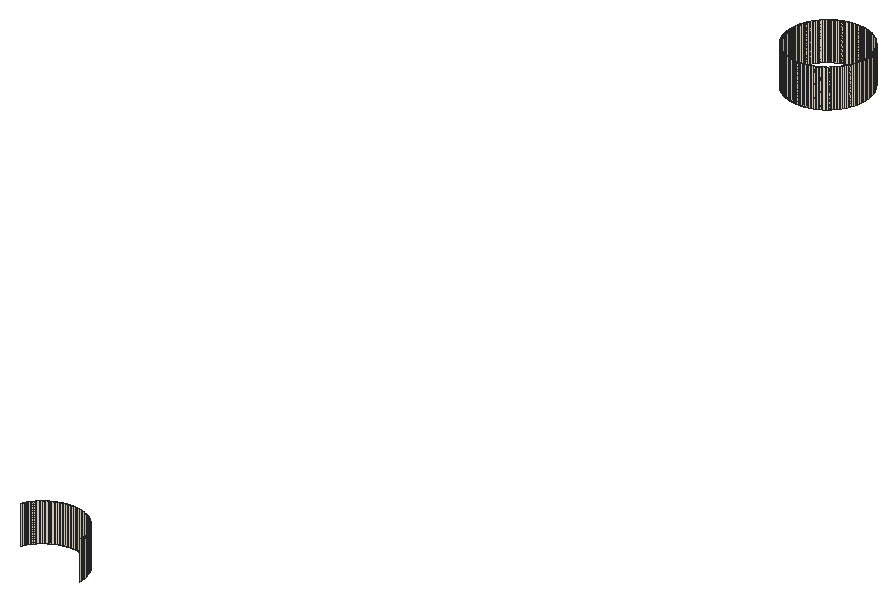
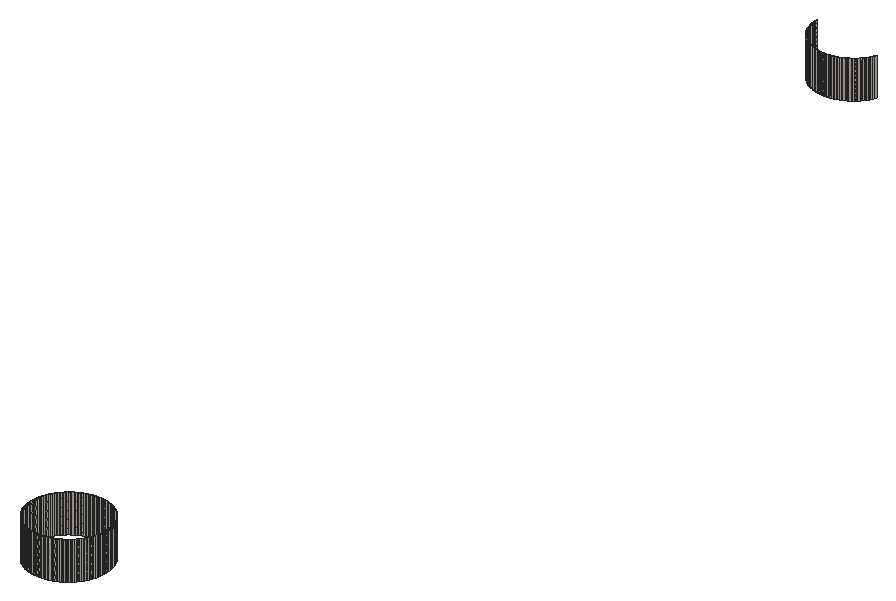
# SketchUp Ruby script. Lengths in inches.
U = 1.inch
M = Sketchup.active_model
def pt(a) = Geom::Point3d.new(a.map { |v| v * U })
def face(e, loops, mat)
  f = e.add_face(loops[0].map { |a| pt(a) })
  loops[1..].each { |l| e.add_face(l.map { |a| pt(a) }).erase! }
  f.material = f.back_material = mat if mat
  f
end
# faces: each face lists its corners as indices into pts; further lists are holes
def faces(e, pts, list, mat = nil) = list.each { |f| face(e, (f[0].is_a?(Array) ? f : [f]).map { |l| l.map { |i| pts[i] } }, mat) }
# xy, xz, yz: faces in a plane at the given z, y or x. An outline is a flat list of corners, or four numbers for a rectangle; further outlines are holes
def ring(l) = l.size == 4 ? [[l[0], l[1]], [l[2], l[1]], [l[2], l[3]], [l[0], l[3]]] : l.each_slice(2).to_a
def flat(e, list, mat, &to3) = list.each { |f| face(e, (f[0].is_a?(Array) ? f : [f]).map { |l| ring(l).map { |u, v| to3.(u, v) } }, mat) }
def xy(e, z, list, mat = nil) = flat(e, list, mat) { |x, y| [x, y, z] }
def xz(e, y, list, mat = nil) = flat(e, list, mat) { |x, z| [x, y, z] }
def yz(e, x, list, mat = nil) = flat(e, list, mat) { |y, z| [x, y, z] }
def lines(e, pts, list) = list.each { |a, b| e.add_line(pt(pts[a]), pt(pts[b])) }
# prism: a flat outline (further loops are holes) pulled along v
def prism(e, loops, v, mat = nil)
  f = face(e, loops, mat); d = Geom::Vector3d.new(v.map { |x| x * U })
  f.pushpull(f.normal.samedirection?(d) ? d.length : -d.length)
end
def box(e, o, s, mat = nil) = prism(e, [[o, [o[0] + s[0], o[1], o[2]], [o[0] + s[0], o[1] + s[1], o[2]], [o[0], o[1] + s[1], o[2]]]], [0, 0, s[2]], mat)
def at(x, y, z, deg = 0) = Geom::Transformation.translation(pt([x, y, z])) * Geom::Transformation.rotation(ORIGIN, Z_AXIS, deg.degrees)
def axes(o, x, y, z) = Geom::Transformation.new([*x, 0, *y, 0, *z, 0, *pt(o).to_a, 1])
def part(name) = M.definitions.add(name)
# library, detail: a bought-in or finely detailed component or shape, given as its bounding box
def library(name, o, s) = part(name).tap { |d| box(d.entities, o, s) }
def detail(e, o, s) = box(e.add_group.entities, o, s)
def put(e, d, t, mat = nil) = e.add_instance(d, t).tap { |i| i.material = mat if mat }
def group(e, t, mat = nil) = e.add_group.tap { |g| g.transformation = t; g.material = mat if mat }.entities
root = M.entities
M.materials.add("0027 AP L140 CRUSHED ICE").color = [241, 233, 217]
xz(root,339,[[122.84,120,122.92,123],[122.92,120,123,123],[123,120,123.08,123],[123.08,120,123.16,123]],"0027 AP L140 CRUSHED ICE")
xz(root,411,[[122.84,120,122.92,123],[122.92,120,123,123],[123,120,123.08,123],[123.08,120,123.16,123]],"0027 AP L140 CRUSHED ICE")
xz(root,417,[[122.84,120,122.92,123],[122.92,120,123,123],[123,120,123.08,123],[123.08,120,123.16,123]],"0027 AP L140 CRUSHED ICE")
yz(root,120,[[413.84,120,413.92,123],[413.92,120,414,123],[414,120,414.08,123],[414.08,120,414.16,123]],"0027 AP L140 CRUSHED ICE")
yz(root,126,[[336,120,336.08,123],[336.08,120,336.16,123],[413.84,120,413.92,123],[413.92,120,414,123],[414.08,120,414.16,123]],"0027 AP L140 CRUSHED ICE")
p = [[125.98,336.3125,120],[125.99,336.24,120],[125.99,336.24,123],[125.98,336.3125,123],[126,336.16,120],[126,336.16,123],
  [125.97,336.39,120],[125.97,336.39,123],[125.96,336.47,120],[125.96,336.47,123],[125.93,336.625,120],[125.95,336.55,120],
  [125.95,336.55,123],[125.93,336.625,123],[125.92,336.7,120],[125.92,336.7,123],[125.9,336.78,120],[125.9,336.78,123],
  [125.875,336.85,120],[125.875,336.85,123],[125.83,337,120],[125.85,336.93,120],[125.85,336.93,123],[125.83,337,123],
  [125.8,337.08,120],[125.8,337.08,123],[125.74,337.22,120],[125.77,337.15,120],[125.77,337.15,123],[125.74,337.22,123],
  [120.26,337.22,120],[120.29,337.29,120],[120.29,337.29,123],[120.26,337.22,123],[125.71,337.29,120],[125.71,337.29,123],
  [120.33,337.36,120],[120.33,337.36,123],[125.67,337.36,120],[125.67,337.36,123],[120.36,337.43,120],[120.36,337.43,123],
  [120.4,337.5,120],[120.4,337.5,123],[125.6,337.5,120],[125.64,337.43,120],[125.64,337.43,123],[125.6,337.5,123],
  [120.44,337.57,120],[120.44,337.57,123],[125.56,337.57,120],[125.56,337.57,123],[120.48,337.63,120],[120.48,337.63,123],
  [120.53,337.7,120],[120.53,337.7,123],[125.47,337.7,120],[125.52,337.63,120],[125.52,337.63,123],[125.47,337.7,123],
  [120.57,337.76,120],[120.57,337.76,123],[125.43,337.76,120],[125.43,337.76,123],[120.62,337.83,120],[120.62,337.83,123],
  [120.67,337.89,120],[120.67,337.89,123],[125.33,337.89,120],[125.38,337.83,120],[125.38,337.83,123],[125.33,337.89,123],
  [120.72,337.95,120],[120.72,337.95,123],[120.77,338.01,120],[120.77,338.01,123],[125.23,338.01,120],[125.28,337.95,120],
  [125.28,337.95,123],[125.23,338.01,123],[120.82,338.07,120],[120.82,338.07,123],[125.18,338.07,120],[125.18,338.07,123],
  [120.88,338.12,120],[120.88,338.12,123],[120.93,338.18,120],[120.93,338.18,123],[125.07,338.18,120],[125.12,338.12,120],
  [125.12,338.12,123],[125.07,338.18,123],[120.99,338.23,120],[120.99,338.23,123],[121.05,338.28,120],[121.05,338.28,123],
  [124.95,338.28,120],[125.01,338.23,120],[125.01,338.23,123],[124.95,338.28,123],[121.11,338.33,120],[121.11,338.33,123],
  [121.17,338.38,120],[121.17,338.38,123],[124.83,338.38,120],[124.89,338.33,120],[124.89,338.33,123],[124.83,338.38,123],
  [121.24,338.43,120],[121.24,338.43,123],[121.3,338.47,120],[121.3,338.47,123],[124.7,338.47,120],[124.76,338.43,120],
  [124.76,338.43,123],[124.7,338.47,123],[121.37,338.52,120],[121.37,338.52,123],[121.43,338.56,120],[121.43,338.56,123],
  [124.57,338.56,120],[124.63,338.52,120],[124.63,338.52,123],[124.57,338.56,123],[121.5,338.6,120],[121.5,338.6,123],
  [121.57,338.64,120],[121.57,338.64,123],[121.64,338.67,120],[121.64,338.67,123],[124.36,338.67,120],[124.43,338.64,120],
  [124.43,338.64,123],[124.36,338.67,123],[124.5,338.6,120],[124.5,338.6,123],[121.71,338.71,120],[121.71,338.71,123],
  [121.78,338.74,120],[121.78,338.74,123],[121.85,338.77,120],[121.85,338.77,123],[124.15,338.77,120],[124.22,338.74,120],
  [124.22,338.74,123],[124.15,338.77,123],[124.29,338.71,120],[124.29,338.71,123],[121.92,338.8,120],[121.92,338.8,123],
  [122,338.83,120],[122,338.83,123],[122.07,338.85,120],[122.07,338.85,123],[123.93,338.85,120],[124,338.83,120],
  [124,338.83,123],[123.93,338.85,123],[124.08,338.8,120],[124.08,338.8,123],[122.15,338.875,120],[122.15,338.875,123],
  [122.22,338.9,120],[122.22,338.9,123],[122.3,338.92,120],[122.3,338.92,123],[122.375,338.93,120],[122.375,338.93,123],
  [122.45,338.95,120],[122.45,338.95,123],[122.53,338.96,120],[122.53,338.96,123],[123.47,338.96,120],[123.55,338.95,120],
  [123.55,338.95,123],[123.47,338.96,123],[123.625,338.93,120],[123.625,338.93,123],[123.7,338.92,120],[123.7,338.92,123],
  [123.78,338.9,120],[123.78,338.9,123],[123.85,338.875,120],[123.85,338.875,123],[122.61,338.97,120],[122.61,338.97,123],
  [122.6875,338.98,120],[122.6875,338.98,123],[122.76,338.99,120],[122.76,338.99,123],[122.84,339,120],[122.84,339,123],
  [123.16,339,120],[123.24,338.99,120],[123.24,338.99,123],[123.16,339,123],[123.3125,338.98,120],[123.3125,338.98,123],
  [123.39,338.97,120],[123.39,338.97,123],[122.61,411.03,120],[122.53,411.04,120],[122.53,411.04,123],[122.61,411.03,123],
  [122.45,411.05,120],[122.45,411.05,123],[122.6875,411.02,120],[122.6875,411.02,123],[122.76,411.01,120],[122.76,411.01,123],
  [122.84,411,120],[122.84,411,123],[123.3125,411.02,120],[123.24,411.01,120],[123.24,411.01,123],[123.3125,411.02,123],
  [123.16,411,120],[123.16,411,123],[123.39,411.03,120],[123.39,411.03,123],[123.47,411.04,120],[123.47,411.04,123],
  [123.55,411.05,120],[123.55,411.05,123],[122.07,411.15,120],[122,411.17,120],[122,411.17,123],[122.07,411.15,123],
  [122.22,411.1,120],[122.15,411.125,120],[122.15,411.125,123],[122.22,411.1,123],[122.3,411.08,120],[122.3,411.08,123],
  [122.375,411.07,120],[122.375,411.07,123],[123.625,411.07,120],[123.625,411.07,123],[123.7,411.08,120],[123.7,411.08,123],
  [123.78,411.1,120],[123.78,411.1,123],[123.85,411.125,120],[123.85,411.125,123],[124,411.17,120],[123.93,411.15,120],
  [123.93,411.15,123],[124,411.17,123],[121.85,411.23,120],[121.78,411.26,120],[121.78,411.26,123],[121.85,411.23,123],
  [121.92,411.2,120],[121.92,411.2,123],[124.08,411.2,120],[124.08,411.2,123],[124.22,411.26,120],[124.15,411.23,120],
  [124.15,411.23,123],[124.22,411.26,123],[121.71,411.29,120],[121.64,411.33,120],[121.64,411.33,123],[121.71,411.29,123],
  [121.57,411.36,120],[121.57,411.36,123],[124.29,411.29,120],[124.29,411.29,123],[124.36,411.33,120],[124.36,411.33,123],
  [124.43,411.36,120],[124.43,411.36,123],[121.5,411.4,120],[121.43,411.44,120],[121.43,411.44,123],[121.5,411.4,123],
  [121.37,411.48,120],[121.37,411.48,123],[124.5,411.4,120],[124.5,411.4,123],[124.57,411.44,120],[124.57,411.44,123],
  [124.63,411.48,120],[124.63,411.48,123],[121.3,411.53,120],[121.24,411.57,120],[121.24,411.57,123],[121.3,411.53,123],
  [124.7,411.53,120],[124.7,411.53,123],[124.76,411.57,120],[124.76,411.57,123],[121.17,411.62,120],[121.11,411.67,120],
  [121.11,411.67,123],[121.17,411.62,123],[124.89,411.67,120],[124.83,411.62,120],[124.83,411.62,123],[124.89,411.67,123],
  [121.05,411.72,120],[120.99,411.77,120],[120.99,411.77,123],[121.05,411.72,123],[125.01,411.77,120],[124.95,411.72,120],
  [124.95,411.72,123],[125.01,411.77,123],[120.93,411.82,120],[120.93,411.82,123],[120.88,411.88,120],[120.88,411.88,123],
  [125.07,411.82,120],[125.07,411.82,123],[125.12,411.88,120],[125.12,411.88,123],[120.82,411.93,120],[120.82,411.93,123],
  [120.77,411.99,120],[120.77,411.99,123],[125.18,411.93,120],[125.18,411.93,123],[125.23,411.99,120],[125.23,411.99,123],
  [120.72,412.05,120],[120.72,412.05,123],[125.28,412.05,120],[125.28,412.05,123],[120.67,412.11,120],[120.62,412.17,120],
  [120.62,412.17,123],[120.67,412.11,123],[125.38,412.17,120],[125.33,412.11,120],[125.33,412.11,123],[125.38,412.17,123],
  [120.57,412.24,120],[120.53,412.3,120],[120.53,412.3,123],[120.57,412.24,123],[125.47,412.3,120],[125.43,412.24,120],
  [125.43,412.24,123],[125.47,412.3,123],[120.48,412.37,120],[120.48,412.37,123],[125.52,412.37,120],[125.52,412.37,123],
  [120.44,412.43,120],[120.44,412.43,123],[120.4,412.5,120],[120.4,412.5,123],[125.56,412.43,120],[125.56,412.43,123],
  [125.6,412.5,120],[125.6,412.5,123],[120.36,412.57,120],[120.36,412.57,123],[125.64,412.57,120],[125.64,412.57,123],
  [120.33,412.64,120],[120.33,412.64,123],[120.29,412.71,120],[120.29,412.71,123],[125.67,412.64,120],[125.67,412.64,123],
  [125.71,412.71,120],[125.71,412.71,123],[120.26,412.78,120],[120.26,412.78,123],[125.74,412.78,120],[125.74,412.78,123],
  [120.23,412.85,120],[120.23,412.85,123],[125.77,412.85,120],[125.77,412.85,123],[120.2,412.92,120],[120.2,412.92,123],
  [120.17,413,120],[120.17,413,123],[125.83,413,120],[125.8,412.92,120],[125.8,412.92,123],[125.83,413,123],
  [120.15,413.07,120],[120.15,413.07,123],[125.85,413.07,120],[125.85,413.07,123],[120.125,413.15,120],[120.125,413.15,123],
  [120.1,413.22,120],[120.1,413.22,123],[125.9,413.22,120],[125.875,413.15,120],[125.875,413.15,123],[125.9,413.22,123],
  [120.08,413.3,120],[120.08,413.3,123],[125.92,413.3,120],[125.92,413.3,123],[120.07,413.375,120],[120.07,413.375,123],
  [125.93,413.375,120],[125.93,413.375,123],[120.05,413.45,120],[120.05,413.45,123],[125.95,413.45,120],[125.95,413.45,123],
  [120.04,413.53,120],[120.04,413.53,123],[120.03,413.61,120],[120.03,413.61,123],[125.96,413.53,120],[125.96,413.53,123],
  [125.97,413.61,120],[125.97,413.61,123],[120.02,413.6875,120],[120.02,413.6875,123],[125.98,413.6875,120],[125.98,413.6875,123],
  [120.01,413.76,120],[120.01,413.76,123],[125.99,413.76,120],[125.99,413.76,123],[120,413.84,120],[120,413.84,123],
  [126,413.84,120],[126,413.84,123],[120,414.16,120],[120.01,414.24,120],[120.01,414.24,123],[120,414.16,123],
  [120.02,414.3125,120],[120.02,414.3125,123],[125.98,414.3125,120],[125.99,414.24,120],[125.99,414.24,123],[125.98,414.3125,123],
  [126,414.16,120],[126,414.16,123],[120.03,414.39,120],[120.03,414.39,123],[125.97,414.39,120],[125.97,414.39,123],
  [120.04,414.47,120],[120.04,414.47,123],[125.96,414.47,120],[125.96,414.47,123],[120.05,414.55,120],[120.05,414.55,123],
  [120.07,414.625,120],[120.07,414.625,123],[125.93,414.625,120],[125.95,414.55,120],[125.95,414.55,123],[125.93,414.625,123],
  [120.08,414.7,120],[120.08,414.7,123],[125.92,414.7,120],[125.92,414.7,123],[120.1,414.78,120],[120.1,414.78,123],
  [125.9,414.78,120],[125.9,414.78,123],[120.125,414.85,120],[120.125,414.85,123],[125.875,414.85,120],[125.875,414.85,123],
  [120.15,414.93,120],[120.15,414.93,123],[120.17,415,120],[120.17,415,123],[125.83,415,120],[125.85,414.93,120],
  [125.85,414.93,123],[125.83,415,123],[120.2,415.08,120],[120.2,415.08,123],[125.8,415.08,120],[125.8,415.08,123],
  [120.23,415.15,120],[120.23,415.15,123],[120.26,415.22,120],[120.26,415.22,123],[125.74,415.22,120],[125.77,415.15,120],
  [125.77,415.15,123],[125.74,415.22,123],[120.29,415.29,120],[120.29,415.29,123],[125.71,415.29,120],[125.71,415.29,123],
  [120.33,415.36,120],[120.33,415.36,123],[125.67,415.36,120],[125.67,415.36,123],[120.36,415.43,120],[120.36,415.43,123],
  [120.4,415.5,120],[120.4,415.5,123],[125.6,415.5,120],[125.64,415.43,120],[125.64,415.43,123],[125.6,415.5,123],
  [120.44,415.57,120],[120.44,415.57,123],[125.56,415.57,120],[125.56,415.57,123],[120.48,415.63,120],[120.48,415.63,123],
  [120.53,415.7,120],[120.53,415.7,123],[125.47,415.7,120],[125.52,415.63,120],[125.52,415.63,123],[125.47,415.7,123],
  [120.57,415.76,120],[120.57,415.76,123],[125.43,415.76,120],[125.43,415.76,123],[120.62,415.83,120],[120.62,415.83,123],
  [120.67,415.89,120],[120.67,415.89,123],[125.33,415.89,120],[125.38,415.83,120],[125.38,415.83,123],[125.33,415.89,123],
  [120.72,415.95,120],[120.72,415.95,123],[120.77,416.01,120],[120.77,416.01,123],[125.23,416.01,120],[125.28,415.95,120],
  [125.28,415.95,123],[125.23,416.01,123],[120.82,416.07,120],[120.82,416.07,123],[125.18,416.07,120],[125.18,416.07,123],
  [120.88,416.12,120],[120.88,416.12,123],[120.93,416.18,120],[120.93,416.18,123],[125.07,416.18,120],[125.12,416.12,120],
  [125.12,416.12,123],[125.07,416.18,123],[120.99,416.23,120],[120.99,416.23,123],[121.05,416.28,120],[121.05,416.28,123],
  [124.95,416.28,120],[125.01,416.23,120],[125.01,416.23,123],[124.95,416.28,123],[121.11,416.33,120],[121.11,416.33,123],
  [121.17,416.38,120],[121.17,416.38,123],[124.83,416.38,120],[124.89,416.33,120],[124.89,416.33,123],[124.83,416.38,123],
  [121.24,416.43,120],[121.24,416.43,123],[121.3,416.47,120],[121.3,416.47,123],[124.7,416.47,120],[124.76,416.43,120],
  [124.76,416.43,123],[124.7,416.47,123],[121.37,416.52,120],[121.37,416.52,123],[121.43,416.56,120],[121.43,416.56,123],
  [124.57,416.56,120],[124.63,416.52,120],[124.63,416.52,123],[124.57,416.56,123],[121.5,416.6,120],[121.5,416.6,123],
  [121.57,416.64,120],[121.57,416.64,123],[121.64,416.67,120],[121.64,416.67,123],[124.36,416.67,120],[124.43,416.64,120],
  [124.43,416.64,123],[124.36,416.67,123],[124.5,416.6,120],[124.5,416.6,123],[121.71,416.71,120],[121.71,416.71,123],
  [121.78,416.74,120],[121.78,416.74,123],[121.85,416.77,120],[121.85,416.77,123],[124.15,416.77,120],[124.22,416.74,120],
  [124.22,416.74,123],[124.15,416.77,123],[124.29,416.71,120],[124.29,416.71,123],[121.92,416.8,120],[121.92,416.8,123],
  [122,416.83,120],[122,416.83,123],[122.07,416.85,120],[122.07,416.85,123],[123.93,416.85,120],[124,416.83,120],
  [124,416.83,123],[123.93,416.85,123],[124.08,416.8,120],[124.08,416.8,123],[122.15,416.875,120],[122.15,416.875,123],
  [122.22,416.9,120],[122.22,416.9,123],[122.3,416.92,120],[122.3,416.92,123],[122.375,416.93,120],[122.375,416.93,123],
  [122.45,416.95,120],[122.45,416.95,123],[122.53,416.96,120],[122.53,416.96,123],[123.47,416.96,120],[123.55,416.95,120],
  [123.55,416.95,123],[123.47,416.96,123],[123.625,416.93,120],[123.625,416.93,123],[123.7,416.92,120],[123.7,416.92,123],
  [123.78,416.9,120],[123.78,416.9,123],[123.85,416.875,120],[123.85,416.875,123],[122.61,416.97,120],[122.61,416.97,123],
  [122.6875,416.98,120],[122.6875,416.98,123],[122.76,416.99,120],[122.76,416.99,123],[122.84,417,120],[122.84,417,123],
  [123.16,417,120],[123.24,416.99,120],[123.24,416.99,123],[123.16,417,123],[123.3125,416.98,120],[123.3125,416.98,123],
  [123.39,416.97,120],[123.39,416.97,123]]
faces(root,p,[[0,1,2,3],[1,4,5,2],[6,0,3,7],[8,6,7,9],[10,11,12,13],[11,8,9,12],[14,10,13,15],[16,14,15,17],
  [18,16,17,19],[20,21,22,23],[21,18,19,22],[24,20,23,25],[26,27,28,29],[27,24,25,28],[30,31,32,33],[34,26,29,35],
  [31,36,37,32],[38,34,35,39],[36,40,41,37],[40,42,43,41],[44,45,46,47],[45,38,39,46],[42,48,49,43],[50,44,47,51],
  [48,52,53,49],[52,54,55,53],[56,57,58,59],[57,50,51,58],[54,60,61,55],[62,56,59,63],[60,64,65,61],[64,66,67,65],
  [68,69,70,71],[69,62,63,70],[66,72,73,67],[72,74,75,73],[76,77,78,79],[77,68,71,78],[74,80,81,75],[82,76,79,83],
  [80,84,85,81],[84,86,87,85],[88,89,90,91],[89,82,83,90],[86,92,93,87],[92,94,95,93],[96,97,98,99],[97,88,91,98],
  [94,100,101,95],[100,102,103,101],[104,105,106,107],[105,96,99,106],[102,108,109,103],[108,110,111,109],[112,113,114,115],[113,104,107,114],
  [110,116,117,111],[116,118,119,117],[120,121,122,123],[121,112,115,122],[118,124,125,119],[124,126,127,125],[126,128,129,127],[130,131,132,133],
  [131,134,135,132],[134,120,123,135],[128,136,137,129],[136,138,139,137],[138,140,141,139],[142,143,144,145],[143,146,147,144],[146,130,133,147],
  [140,148,149,141],[148,150,151,149],[150,152,153,151],[154,155,156,157],[155,158,159,156],[158,142,145,159],[152,160,161,153],[160,162,163,161],
  [162,164,165,163],[164,166,167,165],[166,168,169,167],[168,170,171,169],[172,173,174,175],[173,176,177,174],[176,178,179,177],[178,180,181,179],
  [180,182,183,181],[182,154,157,183],[170,184,185,171],[184,186,187,185],[186,188,189,187],[188,190,191,189],[192,193,194,195],[193,196,197,194],
  [196,198,199,197],[198,172,175,199],[200,201,202,203],[201,204,205,202],[206,200,203,207],[208,206,207,209],[210,208,209,211],[212,213,214,215],
  [213,216,217,214],[218,212,215,219],[220,218,219,221],[222,220,221,223],[224,225,226,227],[228,229,230,231],[229,224,227,230],[232,228,231,233],
  [234,232,233,235],[204,234,235,205],[236,222,223,237],[238,236,237,239],[240,238,239,241],[242,240,241,243],[244,245,246,247],[245,242,243,246],
  [248,249,250,251],[225,252,253,226],[252,248,251,253],[254,244,247,255],[256,257,258,259],[257,254,255,258],[260,261,262,263],[261,264,265,262],
  [249,260,263,250],[266,256,259,267],[268,266,267,269],[270,268,269,271],[272,273,274,275],[273,276,277,274],[264,272,275,265],[278,270,271,279],
  [280,278,279,281],[282,280,281,283],[284,285,286,287],[276,284,287,277],[288,282,283,289],[290,288,289,291],[292,293,294,295],[285,292,295,286],
  [296,297,298,299],[297,290,291,298],[300,301,302,303],[293,300,303,294],[304,305,306,307],[305,296,299,306],[301,308,309,302],[308,310,311,309],
  [312,304,307,313],[314,312,313,315],[310,316,317,311],[316,318,319,317],[320,314,315,321],[322,320,321,323],[318,324,325,319],[326,322,323,327],
  [328,329,330,331],[324,328,331,325],[332,333,334,335],[333,326,327,334],[336,337,338,339],[329,336,339,330],[340,341,342,343],[341,332,335,342],
  [337,344,345,338],[346,340,343,347],[344,348,349,345],[348,350,351,349],[352,346,347,353],[354,352,353,355],[350,356,357,351],[358,354,355,359],
  [356,360,361,357],[360,362,363,361],[364,358,359,365],[366,364,365,367],[362,368,369,363],[370,366,367,371],[368,372,373,369],[374,370,371,375],
  [372,376,377,373],[376,378,379,377],[380,381,382,383],[381,374,375,382],[378,384,385,379],[386,380,383,387],[384,388,389,385],[388,390,391,389],
  [392,393,394,395],[393,386,387,394],[390,396,397,391],[398,392,395,399],[396,400,401,397],[402,398,399,403],[400,404,405,401],[406,402,403,407],
  [404,408,409,405],[408,410,411,409],[412,406,407,413],[414,412,413,415],[410,416,417,411],[418,414,415,419],[416,420,421,417],[422,418,419,423],
  [420,424,425,421],[426,422,423,427],[428,429,430,431],[429,432,433,430],[434,435,436,437],[435,438,439,436],[432,440,441,433],[442,434,437,443],
  [440,444,445,441],[446,442,443,447],[444,448,449,445],[448,450,451,449],[452,453,454,455],[453,446,447,454],[450,456,457,451],[458,452,455,459],
  [456,460,461,457],[462,458,459,463],[460,464,465,461],[466,462,463,467],[464,468,469,465],[468,470,471,469],[472,473,474,475],[473,466,467,474],
  [470,476,477,471],[478,472,475,479],[476,480,481,477],[480,482,483,481],[484,485,486,487],[485,478,479,486],[482,488,489,483],[490,484,487,491],
  [488,492,493,489],[494,490,491,495],[492,496,497,493],[496,498,499,497],[500,501,502,503],[501,494,495,502],[498,504,505,499],[506,500,503,507],
  [504,508,509,505],[508,510,511,509],[512,513,514,515],[513,506,507,514],[510,516,517,511],[518,512,515,519],[516,520,521,517],[520,522,523,521],
  [524,525,526,527],[525,518,519,526],[522,528,529,523],[528,530,531,529],[532,533,534,535],[533,524,527,534],[530,536,537,531],[538,532,535,539],
  [536,540,541,537],[540,542,543,541],[544,545,546,547],[545,538,539,546],[542,548,549,543],[548,550,551,549],[552,553,554,555],[553,544,547,554],
  [550,556,557,551],[556,558,559,557],[560,561,562,563],[561,552,555,562],[558,564,565,559],[564,566,567,565],[568,569,570,571],[569,560,563,570],
  [566,572,573,567],[572,574,575,573],[576,577,578,579],[577,568,571,578],[574,580,581,575],[580,582,583,581],[582,584,585,583],[586,587,588,589],
  [587,590,591,588],[590,576,579,591],[584,592,593,585],[592,594,595,593],[594,596,597,595],[598,599,600,601],[599,602,603,600],[602,586,589,603],
  [596,604,605,597],[604,606,607,605],[606,608,609,607],[610,611,612,613],[611,614,615,612],[614,598,601,615],[608,616,617,609],[616,618,619,617],
  [618,620,621,619],[620,622,623,621],[622,624,625,623],[624,626,627,625],[628,629,630,631],[629,632,633,630],[632,634,635,633],[634,636,637,635],
  [636,638,639,637],[638,610,613,639],[626,640,641,627],[640,642,643,641],[642,644,645,643],[644,646,647,645],[648,649,650,651],[649,652,653,650],
  [652,654,655,653],[654,628,631,655]],"0027 AP L140 CRUSHED ICE")
